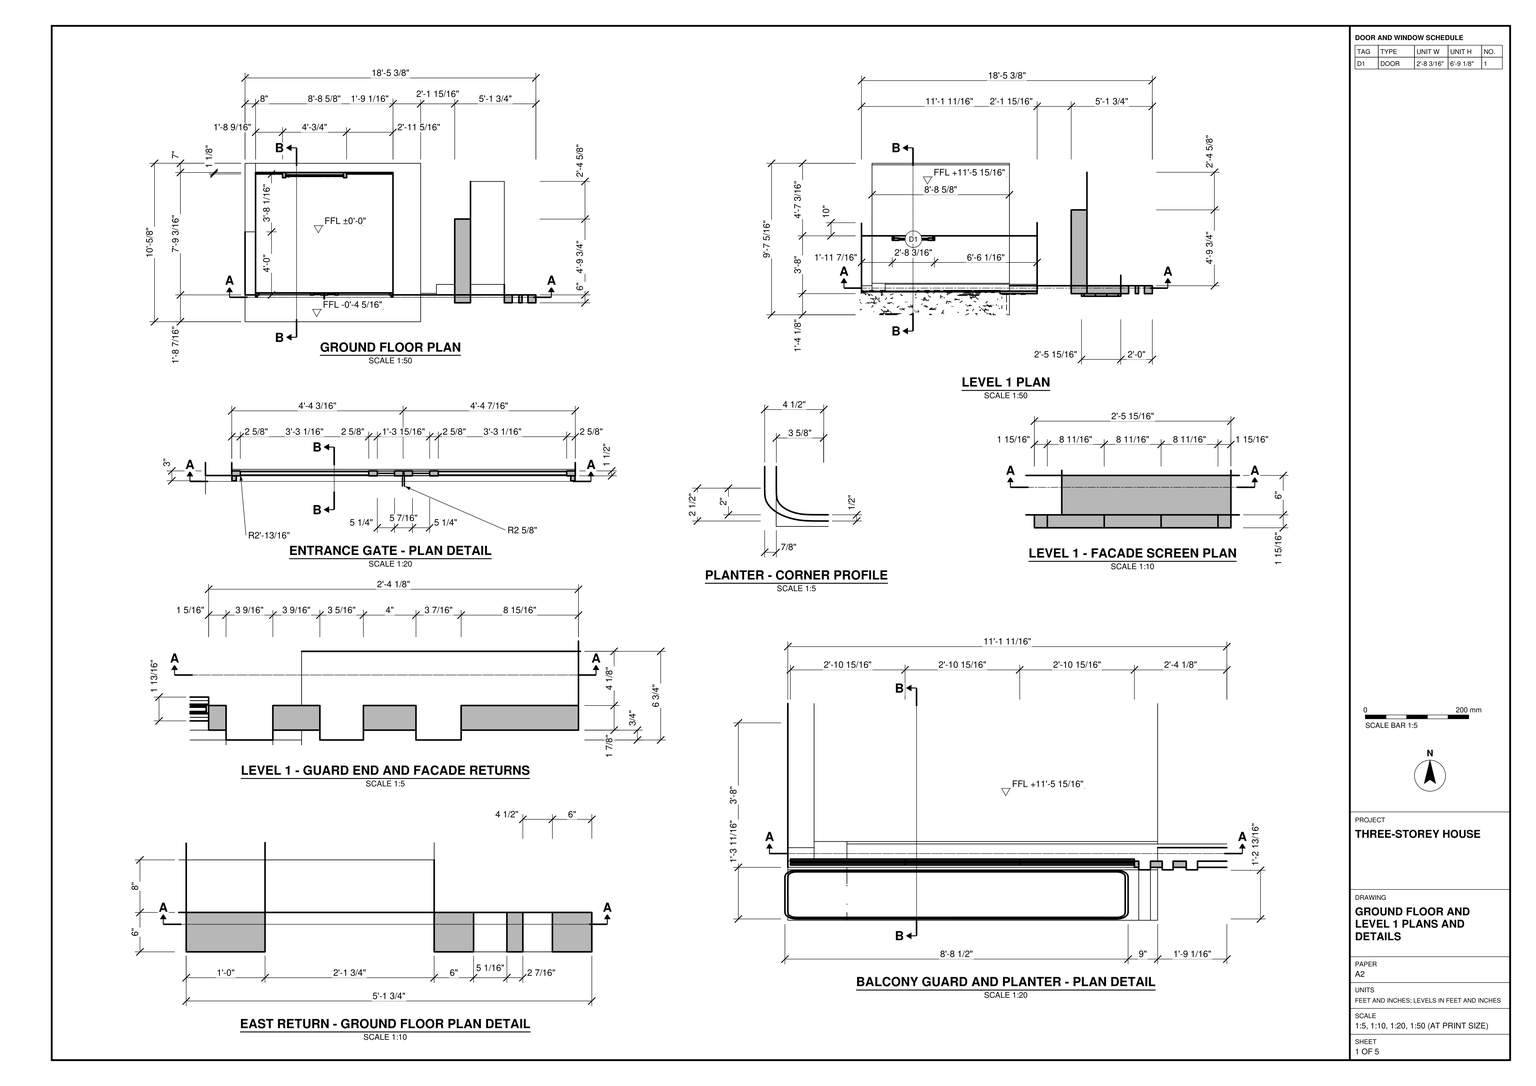
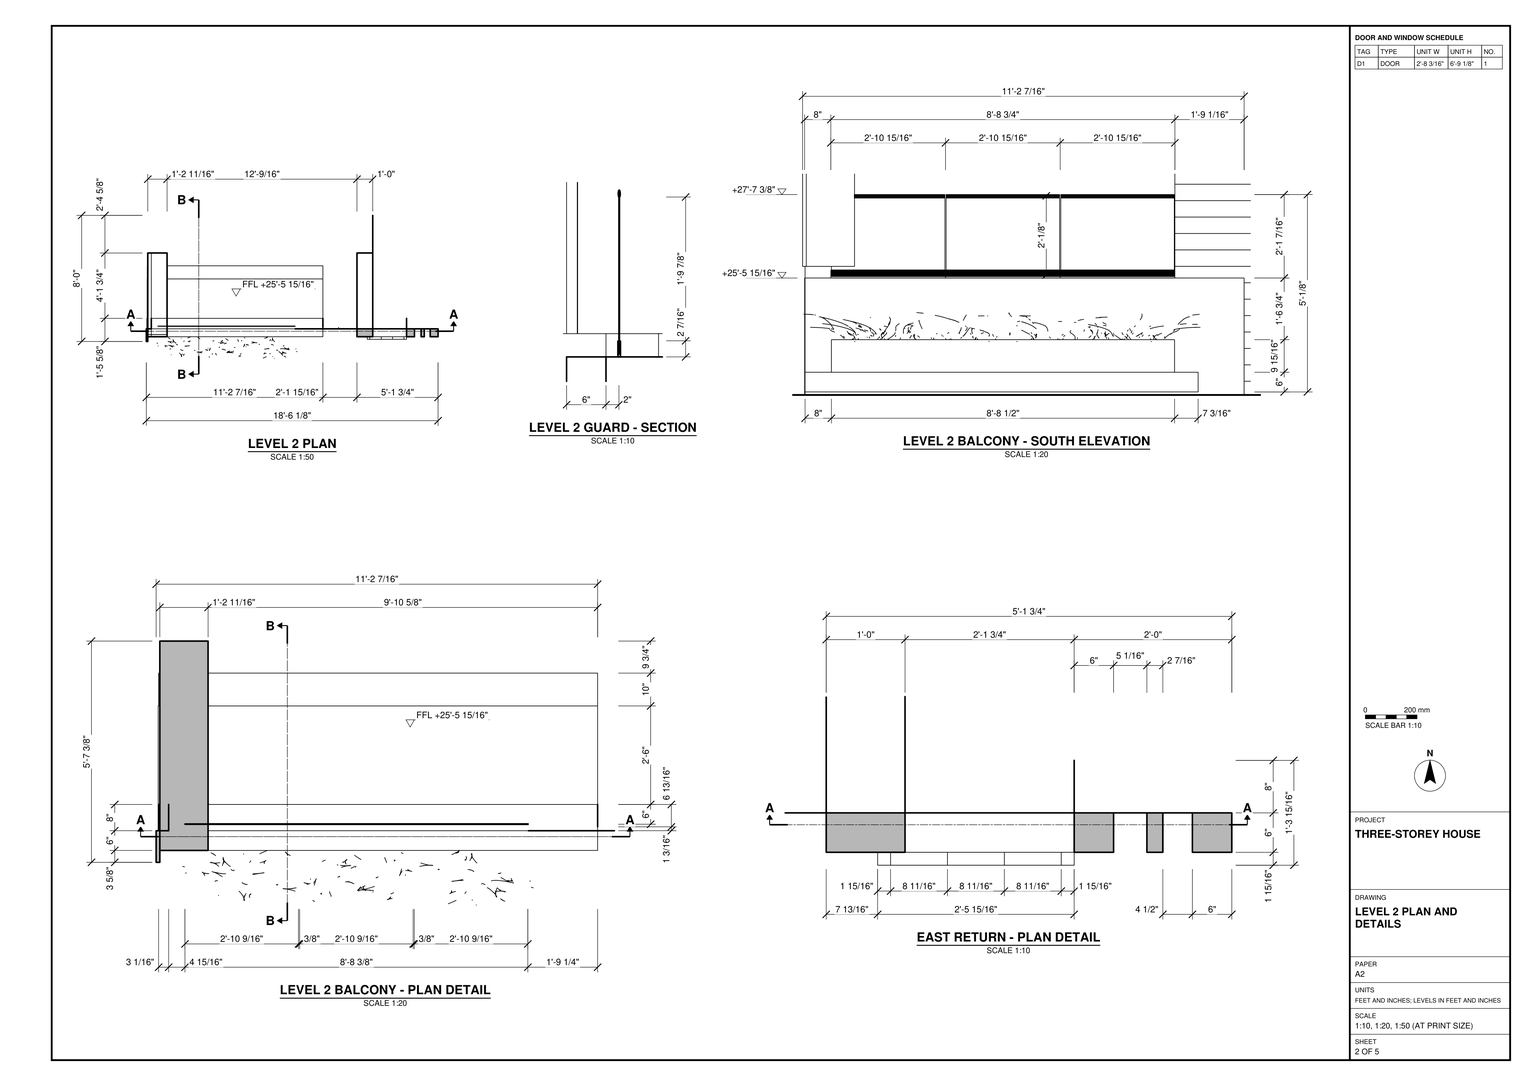
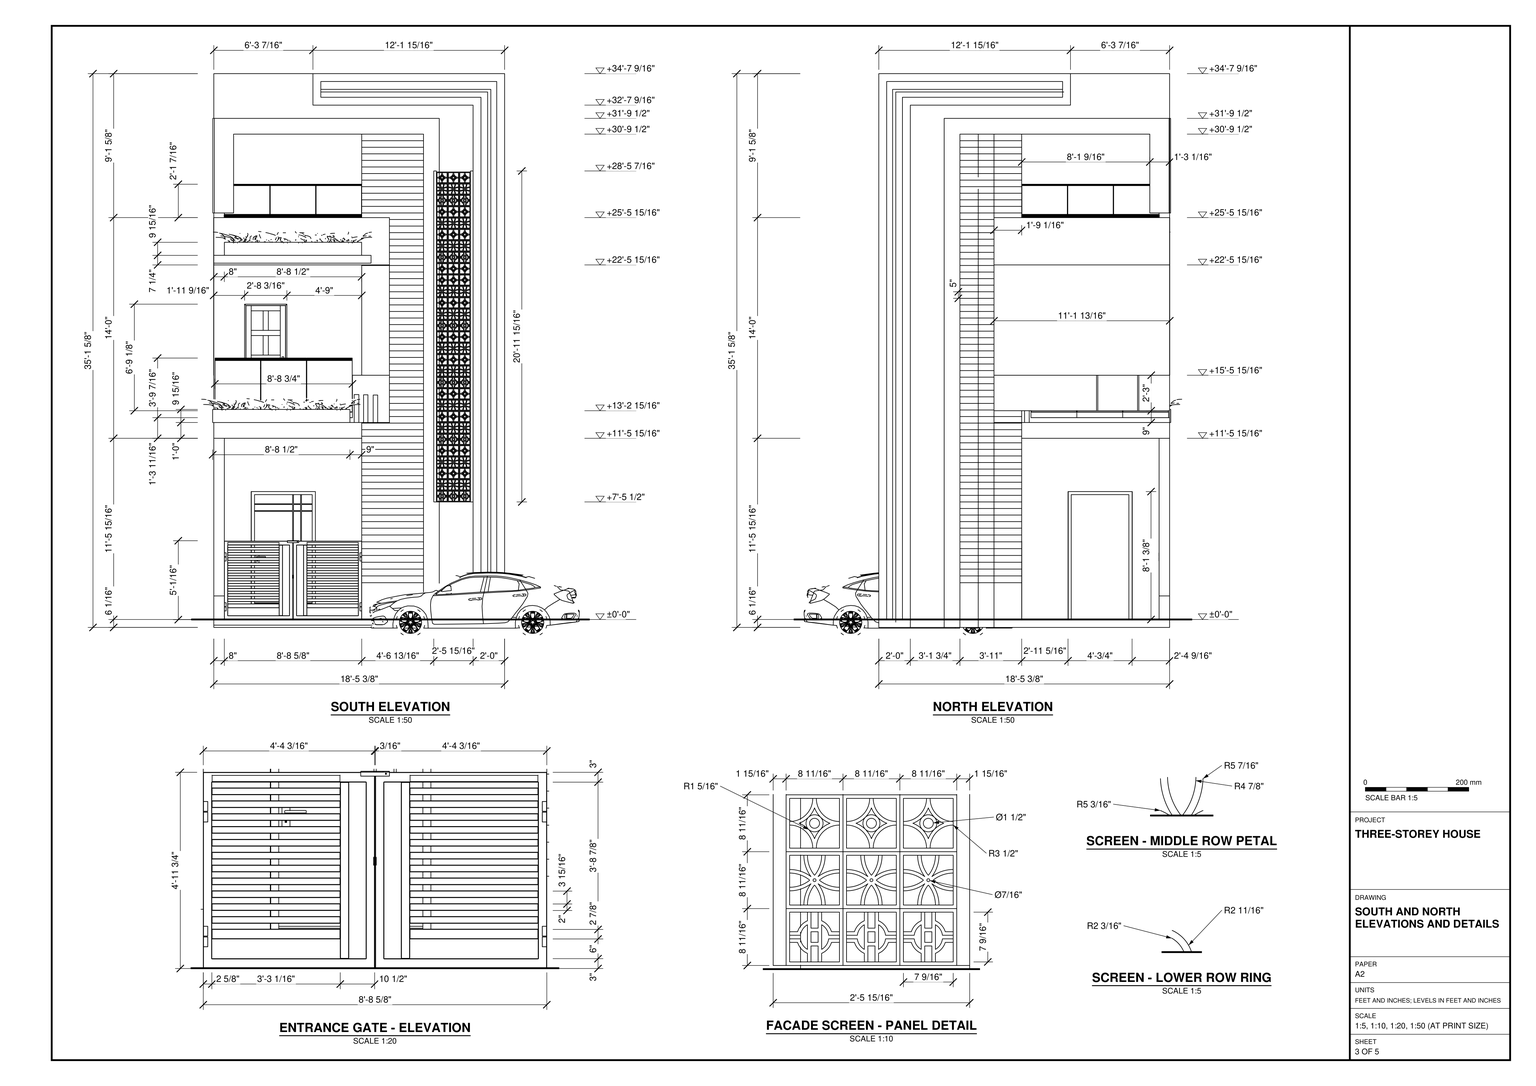
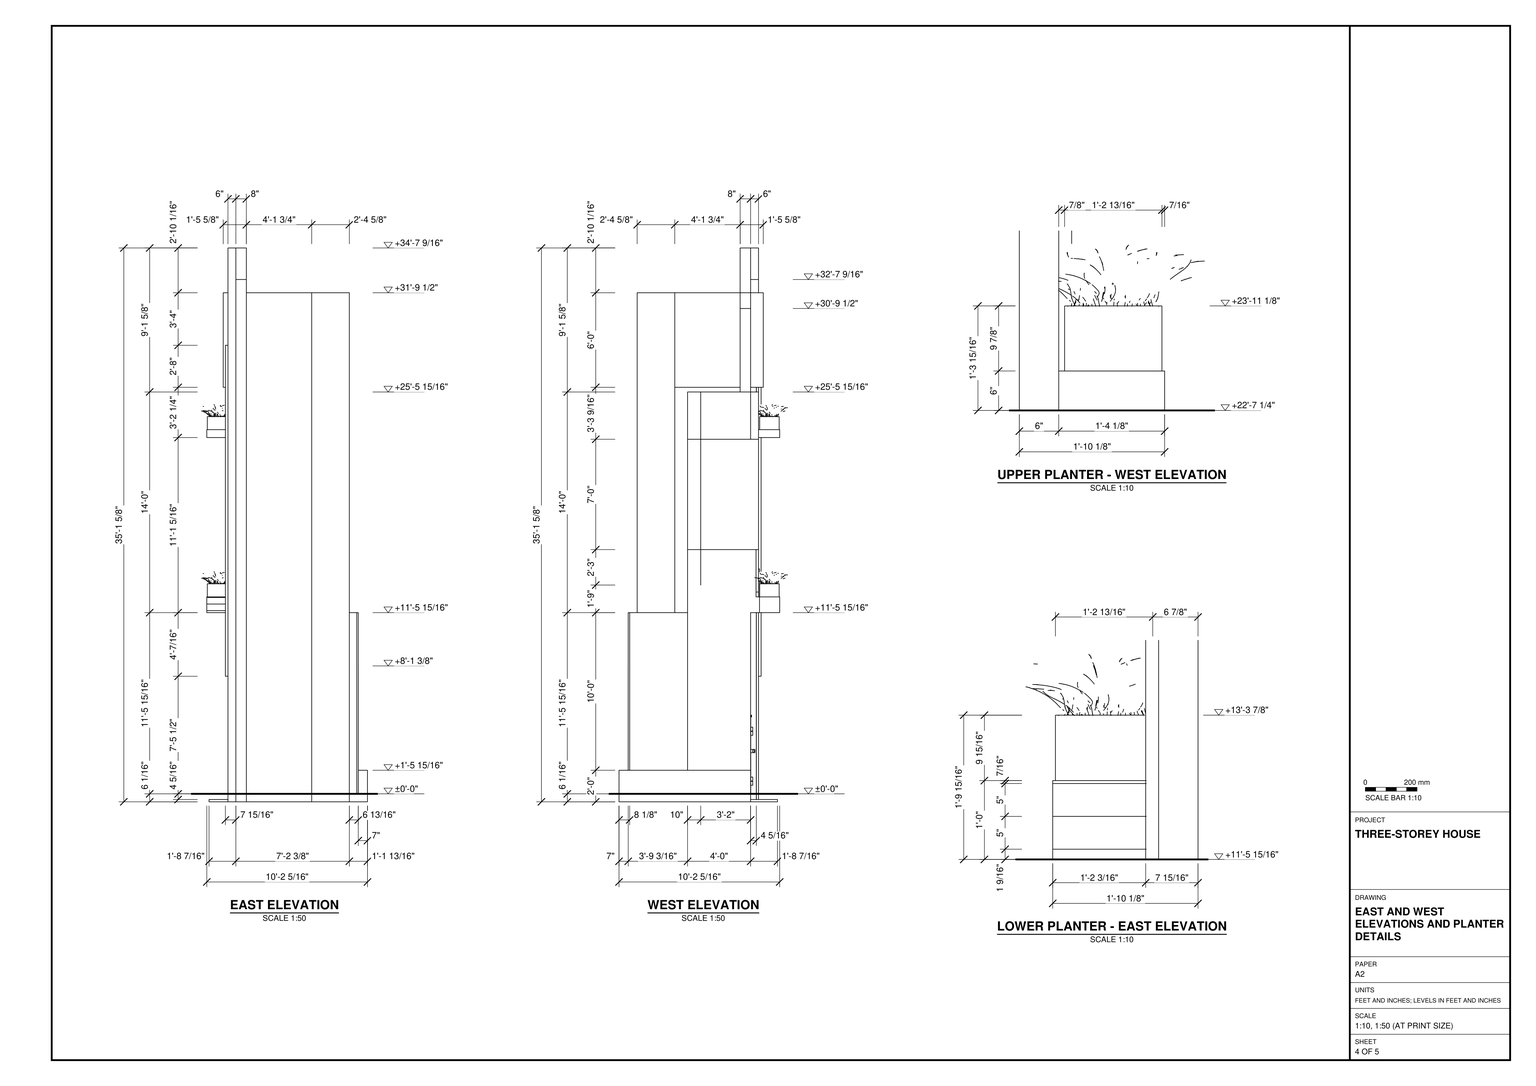
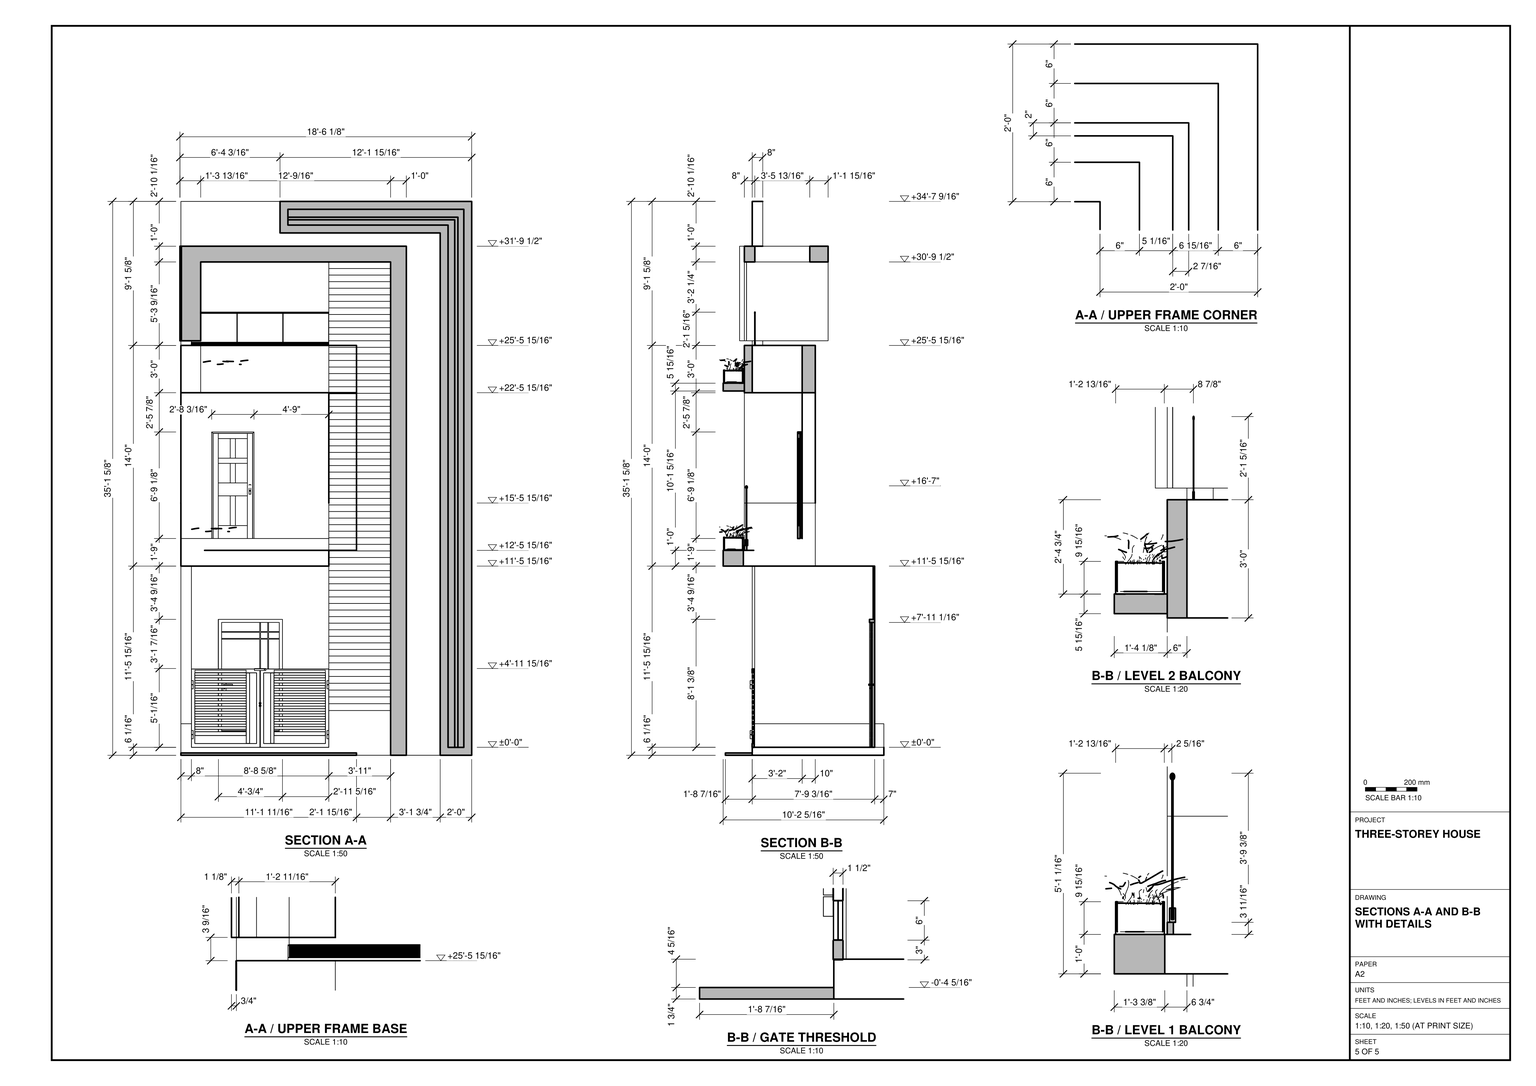
Build the three-storey house frontage in SketchUp from task_files/diagram_01.pdf. Work in feet and inches. The overall model extents, including the parked car, are 24'-11/16" along X, 17'-0" along Y and 35'-8 3/4" along Z. Set the finished floor levels to ±0'-0", +11'-5 15/16" and +25'-5 15/16".

Use the south elevation to lay out the entrance gate and stacked balconies on the left and the tall screened bay on the right. Use the plans and sections to give the walls their drawn thicknesses and to set the depths of the slabs, wall returns and roof-edge framing. Model the two framed, horizontally slatted gate leaves and the opening behind them. Place the scheduled door behind the lower balcony guard. Give both balconies panelled glass guards and projecting planter troughs, following the enlarged details for the guard ends, planter corners and supporting ledges.

Carry the horizontal wall courses alongside the balconies. Build the narrow patterned screen as openwork and continue the stepped outer frame across the top of the façade. Place the car beside the entrance as shown. Decor and loose items, including planting and the car, may be any suitable library components.

Keep walls, slabs, roof elements and individual furniture or joinery pieces in separate groups or components, and use components for repeated parts. Save one SketchUp model as output_files/three_storey_house_facade_with_balconies_and_gate.skp.

# SketchUp Ruby script. Lengths in inches.
U = 1.inch
M = Sketchup.active_model
def pt(a) = Geom::Point3d.new(a.map { |v| v * U })
def face(e, loops, mat)
  f = e.add_face(loops[0].map { |a| pt(a) })
  loops[1..].each { |l| e.add_face(l.map { |a| pt(a) }).erase! }
  f.material = f.back_material = mat if mat
  f
end
# faces: each face lists its corners as indices into pts; further lists are holes
def faces(e, pts, list, mat = nil) = list.each { |f| face(e, (f[0].is_a?(Array) ? f : [f]).map { |l| l.map { |i| pts[i] } }, mat) }
# xy, xz, yz: faces in a plane at the given z, y or x. An outline is a flat list of corners, or four numbers for a rectangle; further outlines are holes
def ring(l) = l.size == 4 ? [[l[0], l[1]], [l[2], l[1]], [l[2], l[3]], [l[0], l[3]]] : l.each_slice(2).to_a
def flat(e, list, mat, &to3) = list.each { |f| face(e, (f[0].is_a?(Array) ? f : [f]).map { |l| ring(l).map { |u, v| to3.(u, v) } }, mat) }
def xy(e, z, list, mat = nil) = flat(e, list, mat) { |x, y| [x, y, z] }
def xz(e, y, list, mat = nil) = flat(e, list, mat) { |x, z| [x, y, z] }
def yz(e, x, list, mat = nil) = flat(e, list, mat) { |y, z| [x, y, z] }
def lines(e, pts, list) = list.each { |a, b| e.add_line(pt(pts[a]), pt(pts[b])) }
# prism: a flat outline (further loops are holes) pulled along v
def prism(e, loops, v, mat = nil)
  f = face(e, loops, mat); d = Geom::Vector3d.new(v.map { |x| x * U })
  f.pushpull(f.normal.samedirection?(d) ? d.length : -d.length)
end
def box(e, o, s, mat = nil) = prism(e, [[o, [o[0] + s[0], o[1], o[2]], [o[0] + s[0], o[1] + s[1], o[2]], [o[0], o[1] + s[1], o[2]]]], [0, 0, s[2]], mat)
def at(x, y, z, deg = 0) = Geom::Transformation.translation(pt([x, y, z])) * Geom::Transformation.rotation(ORIGIN, Z_AXIS, deg.degrees)
def axes(o, x, y, z) = Geom::Transformation.new([*x, 0, *y, 0, *z, 0, *pt(o).to_a, 1])
def part(name) = M.definitions.add(name)
# library, detail: a bought-in or finely detailed component or shape, given as its bounding box
def library(name, o, s) = part(name).tap { |d| box(d.entities, o, s) }
def detail(e, o, s) = box(e.add_group.entities, o, s)
def put(e, d, t, mat = nil) = e.add_instance(d, t).tap { |i| i.material = mat if mat }
def group(e, t, mat = nil) = e.add_group.tap { |g| g.transformation = t; g.material = mat if mat }.entities
root = M.entities
M.materials.add("[0092_Azure]").color = [240, 255, 255]
M.materials.add("[0110_LightSlateGray]").color = [119, 136, 153]
M.materials.add("[0134_DimGray]").color = [105, 105, 105]
M.materials.add("[0135_DarkGray]").color = [81, 81, 81]
M.materials.add("[Cladding Siding Tan]").color = [162, 126, 95]
M.materials.add("[Color D06]").color = [204, 80, 30]
M.materials.add("[Field Square Tile]").color = [217, 201, 169]
M.materials.add("[Tile Limestone Multi]").color = [199, 173, 118]
c1 = library("Residential Interior Door",[0,-1.69,0],[32.2,5.15,81.1])
c2 = library("Untitled",[0,0,0],[36,4.39,84])
c3 = library("T1",[0,0,0],[8.66,8.66,1.97])
c4 = library("T2",[0,0,0],[8.66,8.66,1.97])
c5 = library("T3",[0,0,0],[8.66,8.66,1.97])
c6 = part("1")
box(c6.entities,[-1.97,0,0],[1.97,251.97,1.97],"[0134_DimGray]")
box(c6.entities,[25.98,0,0],[1.97,251.97,1.97],"[0134_DimGray]")
put(c6.entities,c3,at(0,43.31,0),"[Color D06]")
put(c6.entities,c4,at(17.32,25.98,0),"[Color D06]")
put(c6.entities,c5,at(0,34.65,0),"[Color D06]")
put(c6.entities,c4,at(0,8.66,0),"[Color D06]")
put(c6.entities,c5,at(8.66,34.65,0),"[Color D06]")
put(c6.entities,c3,at(8.66,43.31,0),"[Color D06]")
put(c6.entities,c4,at(0,25.98,0),"[Color D06]")
put(c6.entities,c5,at(17.32,34.65,0),"[Color D06]")
put(c6.entities,c4,at(8.66,25.98,0),"[Color D06]")
put(c6.entities,c5,at(17.32,147.24,0),"[Color D06]")
put(c6.entities,c4,at(0,51.97,0),"[Color D06]")
put(c6.entities,c3,at(0,0,0),"[Color D06]")
put(c6.entities,c5,at(8.66,147.24,0),"[Color D06]")
put(c6.entities,c3,at(8.66,0,0),"[Color D06]")
put(c6.entities,c5,at(17.32,17.32,0),"[Color D06]")
put(c6.entities,c4,at(17.32,8.66,0),"[Color D06]")
put(c6.entities,c5,at(8.66,17.32,0),"[Color D06]")
put(c6.entities,c5,at(0,17.32,0),"[Color D06]")
put(c6.entities,c3,at(17.32,0,0),"[Color D06]")
put(c6.entities,c4,at(8.66,8.66,0),"[Color D06]")
put(c6.entities,c3,at(17.32,43.31,0),"[Color D06]")
put(c6.entities,c4,at(8.66,51.97,0),"[Color D06]")
put(c6.entities,c5,at(0,121.26,0),"[Color D06]")
put(c6.entities,c3,at(0,129.92,0),"[Color D06]")
put(c6.entities,c3,at(8.66,129.92,0),"[Color D06]")
put(c6.entities,c4,at(17.32,138.58,0),"[Color D06]")
put(c6.entities,c5,at(0,60.63,0),"[Color D06]")
put(c6.entities,c5,at(8.66,121.26,0),"[Color D06]")
put(c6.entities,c5,at(17.32,121.26,0),"[Color D06]")
put(c6.entities,c4,at(0,112.6,0),"[Color D06]")
put(c6.entities,c4,at(8.66,112.6,0),"[Color D06]")
put(c6.entities,c5,at(8.66,60.63,0),"[Color D06]")
put(c6.entities,c5,at(17.32,60.63,0),"[Color D06]")
put(c6.entities,c4,at(17.32,51.97,0),"[Color D06]")
put(c6.entities,c4,at(17.32,112.6,0),"[Color D06]")
put(c6.entities,c5,at(0,147.24,0),"[Color D06]")
put(c6.entities,c4,at(17.32,69.29,0),"[Color D06]")
put(c6.entities,c5,at(8.66,77.95,0),"[Color D06]")
put(c6.entities,c5,at(0,77.95,0),"[Color D06]")
put(c6.entities,c3,at(8.66,86.61,0),"[Color D06]")
put(c6.entities,c5,at(17.32,77.95,0),"[Color D06]")
put(c6.entities,c4,at(8.66,95.28,0),"[Color D06]")
put(c6.entities,c4,at(8.66,69.29,0),"[Color D06]")
put(c6.entities,c3,at(0,86.61,0),"[Color D06]")
put(c6.entities,c3,at(17.32,86.61,0),"[Color D06]")
put(c6.entities,c5,at(0,103.9375,0),"[Color D06]")
put(c6.entities,c5,at(8.66,103.9375,0),"[Color D06]")
put(c6.entities,c5,at(17.32,103.9375,0),"[Color D06]")
put(c6.entities,c4,at(0,95.28,0),"[Color D06]")
put(c6.entities,c4,at(0,69.29,0),"[Color D06]")
put(c6.entities,c4,at(17.32,95.28,0),"[Color D06]")
put(c6.entities,c5,at(8.66,164.57,0),"[Color D06]")
put(c6.entities,c5,at(0,164.57,0),"[Color D06]")
put(c6.entities,c5,at(17.32,199.21,0),"[Color D06]")
put(c6.entities,c3,at(0,181.89,0),"[Color D06]")
put(c6.entities,c4,at(17.32,190.55,0),"[Color D06]")
put(c6.entities,c3,at(8.66,181.89,0),"[Color D06]")
put(c6.entities,c3,at(17.32,181.89,0),"[Color D06]")
put(c6.entities,c5,at(17.32,164.57,0),"[Color D06]")
put(c6.entities,c5,at(0,199.21,0),"[Color D06]")
put(c6.entities,c5,at(8.66,173.23,0),"[Color D06]")
put(c6.entities,c5,at(8.66,199.21,0),"[Color D06]")
put(c6.entities,c5,at(17.32,173.23,0),"[Color D06]")
put(c6.entities,c4,at(8.66,155.91,0),"[Color D06]")
put(c6.entities,c4,at(0,190.55,0),"[Color D06]")
put(c6.entities,c4,at(8.66,190.55,0),"[Color D06]")
put(c6.entities,c4,at(0,155.91,0),"[Color D06]")
put(c6.entities,c4,at(17.32,155.91,0),"[Color D06]")
put(c6.entities,c5,at(0,173.23,0),"[Color D06]")
put(c6.entities,c4,at(8.66,207.875,0),"[Color D06]")
put(c6.entities,c4,at(0,233.86,0),"[Color D06]")
put(c6.entities,c4,at(8.66,233.86,0),"[Color D06]")
put(c6.entities,c4,at(0,138.58,0),"[Color D06]")
put(c6.entities,c3,at(17.32,129.92,0),"[Color D06]")
put(c6.entities,c5,at(0,216.53,0),"[Color D06]")
put(c6.entities,c3,at(8.66,225.2,0),"[Color D06]")
put(c6.entities,c4,at(17.32,207.875,0),"[Color D06]")
put(c6.entities,c4,at(17.32,233.86,0),"[Color D06]")
put(c6.entities,c5,at(8.66,242.52,0),"[Color D06]")
put(c6.entities,c4,at(0,207.875,0),"[Color D06]")
put(c6.entities,c4,at(8.66,138.58,0),"[Color D06]")
put(c6.entities,c5,at(17.32,216.53,0),"[Color D06]")
put(c6.entities,c5,at(8.66,216.53,0),"[Color D06]")
put(c6.entities,c5,at(17.32,242.52,0),"[Color D06]")
put(c6.entities,c3,at(17.32,225.2,0),"[Color D06]")
put(c6.entities,c5,at(0,242.52,0),"[Color D06]")
put(c6.entities,c3,at(0,225.2,0),"[Color D06]")
c7 = library("2016+Honda+Civic+LX+Sedan",[0.01,0.03,0.02],[16.17,34.46,10.62])
c8 = library("Wagner Glass Railing",[9.08,102.375,1.53],[2.51,145.5,42.05])
c9 = library("Group13",[-203.48,36.63,0],[29.68,67.31,50.64])
c10 = library("Group\#1076",[0,-1.74,0],[119.75,5.32,60.06])
xy(root,16.53,[[0.75,1.6875,134.4375,22.125],[160.375,16.125,172.375,17.75],[198.125,16.125,222.125,22.125],[160.375,17.75,172.375,17.8125],[160.375,17.8125,172.375,22.125],
  [0.75,22.125,134.4375,122.3125],[134.4375,22.125,146.4375,23.3125],[146.4375,22.125,160.375,30.125],[160.375,22.125,172.375,30.125],[172.375,22.125,198.125,30.125],
  [160.375,30.125,172.375,79.875],[172.375,30.125,198.125,108.5]])
xy(root,18.28,[[0.75,1.6875,134.4375,22.125]])
xy(root,22.53,[[204.125,16.125,209.2,22.125],[209.2,16.125,211.625,22.125],[211.625,16.125,216.125,22.125]])
xy(root,22.59,[[8.75,22.125,113.36,24],[8.75,24,113.36,24,113.36,114.1875,77.9,114.1875,77.9,115.3125,29.15,115.3125,29.15,114.1875,8.75,114.1875],[8.75,114.1875,29.15,115.3125],[77.9,114.1875,113.36,115.3125]])
xy(root,40.53,[[0.75,22.125,8.75,70.125],[0.75,70.125,8.75,122.3125]])
xy(root,119.97,[[29.15,114.1875,77.9,115.3125]])
xy(root,160.53,[[0.75,0,8.75,15.375],[8.75,0,18.75,15.375],[18.75,0,113.36,15.375],[0.75,15.375,8.75,22.125],[8.75,15.375,18.75,24],
  [18.75,15.375,113.36,24],[8.75,24,113.36,114.1875],[8.75,114.1875,113.36,115.3125]])
xy(root,172.53,[[0.75,0,18.75,15.375],[18.75,0,107.61,15.375],[107.61,0,111.17,15.375],[111.17,0,113.36,15.375],[0.75,15.375,18.75,16.125],
  [107.61,15.375,111.17,15.375,111.17,18,113.36,18,113.36,22.125,134.4375,22.125,134.4375,23.25,18.75,23.25,18.75,18,107.61,18],[18.75,15.375,107.61,16.125],[111.17,15.375,113.36,16.125],[114.75,15.375,114.75,18,113.36,18,113.36,22.125,134.4375,22.125,134.4375,18,125.5,18,125.5,15.375,122.07,15.375,122.07,18,118.06,18,118.06,15.375],[111.17,16.125,113.36,18],
  [113.36,16.125,114.75,18],[118.06,16.125,122.07,18]])
xy(root,172.53,[[0.75,16.125,18.75,18],[18.75,16.125,107.61,18],[125.5,16.125,134.4375,18]],"[0135_DarkGray]")
xy(root,176.22,[[0.75,16.125,106.28,18]],"[0135_DarkGray]")
xy(root,193.47,[[122.07,15.375,125.5,16.125]],"[0092_Azure]")
xy(root,193.47,[[122.07,16.125,125.5,18]],"[0135_DarkGray]")
xy(root,193.65,[[114.75,15.375,118.06,16.125]],"[0092_Azure]")
xy(root,193.65,[[114.75,16.125,118.06,18]],"[0135_DarkGray]")
xy(root,193.84,[[107.61,15.375,111.17,16.125]],"[0092_Azure]")
xy(root,193.84,[[107.61,16.125,111.17,18]],"[0135_DarkGray]")
xy(root,208.53,[[0.625,16.125,0.625,60.125,0.75,16.125],[0.75,16.125,0.625,60.125,0.75,60.125]])
xy(root,208.53,[[106.28,16.125,113.36,18],[113.36,16.125,134.4375,18]],"[0135_DarkGray]")
xy(root,292.08,[[113.36,16.125,134.4375,22.125]])
xy(root,292.53,[[0.75,16.125,0.73,22.125,0.75,22.125],[0.75,16.125,134.4375,22.125],[0.625,22.125,0.625,60.125,0.73,22.125],[0.75,60.125,134.4375,70.125]])
xy(root,292.53,[[0.73,22.125,0.625,60.125,134.4375,60.125,134.4375,22.125]],"[Field Square Tile]")
xy(root,293.83,[[0.75,0,120.4375,16.125]],"[0092_Azure]")
xy(root,299.83,[[0.75,0,120.4375,16.125]],"[0092_Azure]")
xy(root,328.53,[[0.75,16.125,134.4375,22.125],[0.625,22.125,0.75,22.125,0.75,30.125,15.8125,30.125,15.8125,60.125,0.625,60.125],[0.75,22.125,15.8125,30.125],[15.8125,22.125,134.4375,30.125],[15.8125,30.125,134.4375,60.125],
  [0.75,60.125,134.4375,70.125]])
xy(root,332.07,[[0,12.5,1.125,22.125],[1.125,16.125,3.8125,17.75],[3.8125,16.125,15.8125,17.75],[1.125,17.75,3.8125,17.8125],[3.8125,17.75,15.8125,17.8125],
  [1.125,17.8125,3.8125,22.125],[3.8125,17.8125,15.8125,22.125],[1.125,22.125,3.8125,79.875],[3.8125,22.125,15.8125,30.125],[3.8125,30.125,15.8125,79.875]])
xy(root,392.08,[[15.8125,16.125,18.75,17.75],[[18.75,16.125,18.75,79.875,160.375,79.875,160.375,22.125,146.4375,22.125,146.4375,23.3125,134.4375,23.3125,134.4375,22.125,160.375,22.125,160.375,16.125],[29.05,24.12,43.55,65.93],[50.19,23.69,63.07,65.69]],[15.8125,17.75,18.75,17.8125],[15.8125,17.8125,18.75,22.125],[15.8125,22.125,18.75,30.125],
  [134.4375,22.125,146.4375,23.3125],[134.4375,22.125,146.4375,23.3125],[15.8125,30.125,18.75,79.875]])
xy(root,404.07,[[0,12.5,1.125,22.125],[1.125,16.125,146.4375,17.75],[146.4375,16.125,172.375,17.75],[1.125,17.75,146.4375,17.8125],[146.4375,17.75,172.375,17.8125],
  [1.125,17.8125,146.4375,22.125],[146.4375,17.8125,172.375,22.125],[1.125,22.125,3.8125,79.875],[3.8125,22.125,18.75,30.125],[3.8125,22.125,18.75,79.875],
  [18.75,22.125,146.4375,22.125,146.4375,30.125,63.07,30.125,63.07,23.69,50.19,23.69,50.19,30.125,43.55,30.125,43.55,24.12,29.05,24.12,29.05,30.125,18.75,30.125],[146.4375,22.125,172.375,79.875],[50.19,23.69,63.07,30.125],[29.05,24.12,43.55,30.125],[3.8125,30.125,18.75,79.875],
  [18.75,30.125,29.05,30.125,29.05,65.93,43.55,65.93,43.55,30.125,50.19,30.125,50.19,65.69,63.07,65.69,63.07,30.125,146.4375,30.125,146.4375,79.875,18.75,79.875],[146.4375,79.875,172.375,108.5]])
xy(root,414.15,[[76.22,16.125,198.125,22.125],[76.22,22.125,198.125,30.125]])
xy(root,420.15,[[82.22,16.125,204.125,22.125]],"[0110_LightSlateGray]")
xy(root,424.17,[[82.22,16.125,209.2,22.125]],"[0110_LightSlateGray]")
xy(root,426.15,[[82.22,16.125,211.625,22.125]],"[0110_LightSlateGray]")
xy(root,432.15,[[82.22,16.125,216.125,22.125]])
xy(root,438.15,[[76.22,16.125,222.125,22.125],[0.75,22.125,76.22,30.125]])
xz(root,0,[[0.75,160.53,113.36,172.53]])
xz(root,0,[[0.75,293.83,120.4375,299.83]],"[0092_Azure]")
xz(root,1.6875,[[0.75,16.53,134.4375,18.28]])
xz(root,12.5,[[0,332.07,1.125,404.07]])
xz(root,15.375,[[0.75,160.53,113.36,172.53]])
xz(root,15.375,[[107.61,172.53,111.17,193.84],[114.75,172.53,118.06,193.65],[122.07,172.53,125.5,193.47]],"[0092_Azure]")
xz(root,16.125,[[160.375,16.53,172.375,16.53,172.375,404.07,1.125,404.07,1.125,332.07,15.8125,332.07,15.8125,392.08,160.375,392.08],[209.2,22.53,211.625,22.53,211.625,426.15,82.22,426.15,82.22,424.17,209.2,424.17]])
xz(root,16.125,[[0.75,293.83,120.4375,299.83]],"[0092_Azure]")
xz(root,16.125,[[[198.125,16.53,222.125,16.53,222.125,438.15,76.22,438.15,76.22,414.15,198.125,414.15],[204.125,22.53,204.125,420.15,82.22,420.15,82.22,432.15,216.125,432.15,216.125,22.53]]],"[0110_LightSlateGray]")
xz(root,16.125,[[0.75,172.53,107.61,172.53,107.61,193.84,111.17,193.84,111.17,172.53,114.75,172.53,114.75,193.65,118.06,193.65,118.06,172.53,122.07,172.53,122.07,193.47,125.5,193.47,125.5,172.53,134.4375,172.53,134.4375,208.53,106.28,208.53,106.28,176.22,0.75,176.22],[113.36,208.53,134.4375,292.08],[0.75,292.53,134.4375,292.53,134.4375,328.53,0.75,328.53,0.75,299.83,120.4375,299.83,120.4375,293.83,0.75,293.83]],"[0135_DarkGray]")
xz(root,18,[[0.75,172.53,0.75,176.22,106.28,176.22,106.28,208.53,134.4375,208.53,134.4375,172.53,125.5,172.53,125.5,193.47,122.07,193.47,122.07,172.53,118.06,172.53,118.06,193.65,114.75,193.65,114.75,172.53,111.17,172.53,111.17,193.84,107.61,193.84,107.61,172.53]],"[0135_DarkGray]")
xz(root,22.125,[[0.75,16.53,134.4375,18.28],[134.4375,16.53,160.375,16.53,160.375,50.58,113.36,50.58,113.36,22.59,8.75,22.59,8.75,40.53,0.75,40.53,0.75,18.28,134.4375,18.28],[[198.125,16.53,198.125,414.15,76.22,414.15,76.22,438.15,222.125,438.15,222.125,16.53],[204.125,22.53,216.125,22.53,216.125,432.15,82.22,432.15,82.22,420.15,204.125,420.15]],[160.375,16.53,172.375,16.53,172.375,404.07,146.4375,404.07,146.4375,392.08,160.375,392.08],[209.2,22.53,209.2,424.17,82.22,424.17,82.22,426.15,211.625,426.15,211.625,22.53],
  [0.75,40.53,8.75,160.53],[113.36,50.58,160.375,55.77],[113.36,172.08,134.4375,172.53],[113.36,172.53,134.4375,177.08],[113.36,177.08,134.4375,182.08],
  [113.36,182.08,134.4375,187.08],[113.36,187.08,134.4375,192.08],[113.36,192.08,134.4375,197.08],[113.36,197.08,134.4375,202.08],[113.36,202.08,134.4375,207.08],
  [113.36,207.08,134.4375,212.08],[113.36,212.08,134.4375,217.08],[113.36,217.08,134.4375,222.08],[113.36,222.08,134.4375,227.08],[113.36,227.08,134.4375,232.08],
  [113.36,232.08,134.4375,237.08],[113.36,237.08,134.4375,242.08],[113.36,242.08,134.4375,247.08],[113.36,247.08,134.4375,252.08],[113.36,252.08,134.4375,257.08],
  [113.36,257.08,134.4375,262.08],[113.36,262.08,134.4375,267.08],[113.36,267.08,134.4375,272.08],[113.36,272.08,134.4375,277.08],[113.36,277.08,134.4375,282.08],
  [113.36,282.08,134.4375,287.08],[113.36,287.08,134.4375,292.08],[113.36,292.08,134.4375,292.53],[0.625,292.53,0.75,328.53],[0.75,292.53,15.8125,328.53],
  [15.8125,292.53,113.36,328.53],[113.36,292.53,134.4375,297.08],[113.36,297.08,134.4375,302.08],[113.36,302.08,134.4375,307.08],[113.36,307.08,134.4375,312.08],
  [113.36,312.08,134.4375,317.08],[113.36,317.08,134.4375,322.08],[113.36,322.08,134.4375,327.08],[113.36,327.08,134.4375,328.53],[0,332.07,0.75,404.07],
  [0.75,332.07,1.125,404.07],[1.125,332.07,3.8125,404.07]])
xz(root,22.125,[[204.125,22.53,209.2,22.53,209.2,424.17,82.22,424.17,82.22,420.15,204.125,420.15],[211.625,22.53,216.125,22.53,216.125,432.15,82.22,432.15,82.22,426.15,211.625,426.15]],"[0110_LightSlateGray]")
xz(root,22.125,[[113.36,55.77,160.375,60.96],[113.36,60.96,160.375,66.15],[113.36,66.15,160.375,71.33],[113.36,71.33,160.375,76.52],[113.36,76.52,160.375,81.71],
  [113.36,81.71,160.375,86.9],[113.36,86.9,160.375,92.08],[113.36,92.08,160.375,97.08],[113.36,97.08,160.375,102.08],[113.36,102.08,160.375,107.08],
  [113.36,107.08,160.375,112.08],[113.36,112.08,160.375,117.08],[113.36,117.08,160.375,122.08],[113.36,122.08,160.375,127.08],[113.36,127.08,160.375,132.08],
  [113.36,132.08,160.375,137.08],[113.36,137.08,160.375,142.08],[113.36,142.08,160.375,147.08],[113.36,147.08,160.375,152.08],[113.36,152.08,160.375,157.08],
  [113.36,157.08,160.375,162.08],[113.36,162.08,160.375,167.08],[113.36,167.08,160.375,172.08],[134.4375,172.08,160.375,177.08],[134.4375,177.08,160.375,182.08],
  [134.4375,182.08,160.375,187.08],[134.4375,187.08,160.375,192.08],[134.4375,192.08,160.375,197.08],[134.4375,197.08,160.375,202.08],[134.4375,202.08,160.375,207.08],
  [134.4375,207.08,160.375,212.08],[134.4375,212.08,160.375,217.08],[134.4375,217.08,160.375,222.08],[134.4375,222.08,160.375,227.08],[134.4375,227.08,160.375,232.08],
  [134.4375,232.08,160.375,237.08],[134.4375,237.08,160.375,242.08],[134.4375,242.08,160.375,247.08],[134.4375,247.08,160.375,252.08],[134.4375,252.08,160.375,257.08],
  [134.4375,257.08,160.375,262.08],[134.4375,262.08,160.375,267.08],[134.4375,267.08,160.375,272.08],[134.4375,272.08,160.375,277.08],[134.4375,277.08,160.375,282.08],
  [134.4375,282.08,160.375,287.08],[134.4375,287.08,160.375,292.08],[134.4375,292.08,160.375,297.08],[134.4375,297.08,160.375,302.08],[134.4375,302.08,160.375,307.08],
  [134.4375,307.08,160.375,312.08],[134.4375,312.08,160.375,317.08],[134.4375,317.08,160.375,322.08],[134.4375,322.08,160.375,327.08],[134.4375,327.08,160.375,327.08,160.375,332.08,113.36,332.08,113.36,328.53,134.4375,328.53],
  [113.36,332.08,160.375,337.08],[113.36,337.08,160.375,342.08],[113.36,342.08,160.375,347.08],[113.36,347.08,160.375,352.08],[113.36,352.08,160.375,357.08],
  [113.36,357.08,160.375,362.08],[113.36,362.08,160.375,367.08],[113.36,367.08,160.375,372.08],[113.36,372.08,160.375,377.08],[113.36,377.08,160.375,382.08],
  [113.36,382.08,160.375,387.08],[113.36,387.08,160.375,392.08]],"[Cladding Siding Tan]")
xz(root,22.125,[[172.375,16.53,198.125,16.53,198.125,414.15,76.22,414.15,76.22,438.15,0.75,438.15,0.75,404.07,172.375,404.07]],"[Tile Limestone Multi]")
xz(root,23.69,[[50.19,392.08,63.07,404.07]])
xz(root,24.12,[[29.05,392.08,43.55,404.07]])
xz(root,60.125,[[0.625,208.53,0.75,280.15],[0.625,280.15,0.75,291.09],[0.625,291.09,0.75,292.53],[0.625,292.53,0.75,328.53],[0.75,292.53,15.8125,328.53],
  [15.8125,292.53,134.4375,328.53]])
xz(root,60.125,[[0.75,181.53,134.4375,292.53]],"[Field Square Tile]")
xz(root,65.69,[[50.19,392.08,63.07,404.07]])
xz(root,65.93,[[29.05,392.08,43.55,404.07]])
xz(root,70.125,[[0.75,208.53,134.4375,292.53],[0.75,292.53,134.4375,328.53]])
xz(root,79.875,[[160.375,16.53,160.375,392.08,15.8125,392.08,15.8125,332.07,1.125,332.07,1.125,404.07,172.375,404.07,172.375,16.53]])
xz(root,114.1875,[[8.75,22.59,29.15,22.59,29.15,119.97,77.9,119.97,77.9,22.59,113.36,22.59,113.36,160.53,8.75,160.53]],"[Field Square Tile]")
xz(root,115.3125,[[8.75,22.59,8.75,160.53,113.36,160.53,113.36,22.59,77.9,22.59,77.9,119.97,29.15,119.97,29.15,22.59],[29.15,22.59,77.9,119.97]])
xz(root,122.3125,[[0.75,16.53,0.75,40.53,8.75,40.53,8.75,22.59,134.4375,22.59,134.4375,16.53]])
yz(root,0,[[12.5,332.07,22.125,404.07]])
yz(root,0.625,[[22.125,292.53,60.125,328.53]])
yz(root,0.75,[[1.6875,16.53,22.125,18.28],[22.125,16.53,122.3125,40.53],[22.125,40.53,22.125,160.53,15.375,160.53,15.375,172.53,18,172.53,18,208.53,70.125,208.53,70.125,40.53],[0,160.53,15.375,172.53],[60.125,208.53,70.125,292.53],
  [16.125,292.53,22.125,328.53],[60.125,292.53,70.125,328.53],[22.125,328.53,30.125,392.08],[22.125,392.08,30.125,404.07],[22.125,404.07,30.125,438.15]])
yz(root,0.75,[[0,293.83,16.125,299.83]],"[0092_Azure]")
yz(root,0.75,[[16.125,172.53,18,176.22],[16.125,176.22,18,208.53]],"[0135_DarkGray]")
yz(root,1.125,[[12.5,332.07,16.125,404.07],[16.125,332.07,17.75,404.07],[17.75,332.07,17.8125,404.07],[17.8125,332.07,22.125,404.07],[22.125,332.07,79.875,404.07]])
yz(root,3.8125,[[22.125,332.07,30.125,404.07]])
yz(root,8.75,[[22.125,22.59,24,40.53],[24,22.59,114.1875,40.53],[114.1875,22.59,115.3125,40.53],[115.3125,22.59,122.3125,40.53],[22.125,40.53,24,160.53],
  [114.1875,40.53,115.3125,160.53]])
yz(root,8.75,[[24,40.53,114.1875,160.53]],"[Field Square Tile]")
yz(root,15.8125,[[16.125,332.07,17.75,392.08],[17.75,332.07,17.8125,392.08]])
yz(root,15.8125,[[17.8125,332.07,79.875,392.08]],"[Field Square Tile]")
yz(root,29.05,[[24.12,392.08,65.93,404.07]])
yz(root,29.15,[[114.1875,22.59,115.3125,119.97]])
yz(root,43.55,[[24.12,392.08,65.93,404.07]])
yz(root,50.19,[[23.69,392.08,65.69,404.07]])
yz(root,63.07,[[23.69,392.08,65.69,404.07]])
yz(root,76.22,[[16.125,414.15,22.125,438.15],[22.125,414.15,30.125,438.15]])
yz(root,77.9,[[114.1875,22.59,115.3125,119.97]])
yz(root,82.22,[[16.125,424.17,22.125,426.15]])
yz(root,82.22,[[16.125,420.15,22.125,424.17],[16.125,426.15,22.125,432.15]],"[0110_LightSlateGray]")
yz(root,106.28,[[16.125,176.22,18,208.53]],"[0135_DarkGray]")
yz(root,107.61,[[15.375,172.53,16.125,193.84]],"[0092_Azure]")
yz(root,107.61,[[16.125,172.53,18,193.84]],"[0135_DarkGray]")
yz(root,111.17,[[15.375,172.53,16.125,193.84]],"[0092_Azure]")
yz(root,111.17,[[16.125,172.53,18,193.84]],"[0135_DarkGray]")
yz(root,113.36,[[22.125,22.59,24,50.58],[114.1875,22.59,115.3125,160.53],[22.125,50.58,24,55.77],[22.125,55.77,24,60.96],[22.125,60.96,24,66.15],
  [22.125,66.15,24,71.33],[22.125,71.33,24,76.52],[22.125,76.52,24,81.71],[22.125,81.71,24,86.9],[22.125,86.9,24,92.08],
  [22.125,92.08,24,97.08],[22.125,97.08,24,102.08],[22.125,102.08,24,107.08],[22.125,107.08,24,112.08],[22.125,112.08,24,117.08],
  [22.125,117.08,24,122.08],[22.125,122.08,24,127.08],[22.125,127.08,24,132.08],[22.125,132.08,24,137.08],[22.125,137.08,24,142.08],
  [22.125,142.08,24,147.08],[22.125,147.08,24,152.08],[22.125,152.08,24,157.08],[22.125,157.08,24,160.53],[0,160.53,15.375,162.08],
  [15.375,160.53,22.125,162.08],[0,162.08,15.375,167.08],[15.375,162.08,22.125,167.08],[0,167.08,15.375,172.08],[15.375,167.08,22.125,172.08],
  [0,172.08,15.375,172.53],[15.375,172.08,22.125,172.53]])
yz(root,113.36,[[16.125,208.53,22.125,292.08]],"[0135_DarkGray]")
yz(root,113.36,[[24,22.59,114.1875,160.53]],"[Field Square Tile]")
yz(root,114.75,[[15.375,172.53,16.125,193.65]],"[0092_Azure]")
yz(root,114.75,[[16.125,172.53,18,193.65]],"[0135_DarkGray]")
yz(root,118.06,[[15.375,172.53,16.125,193.65]],"[0092_Azure]")
yz(root,118.06,[[16.125,172.53,18,193.65]],"[0135_DarkGray]")
yz(root,120.4375,[[0,293.83,16.125,299.83]],"[0092_Azure]")
yz(root,122.07,[[15.375,172.53,16.125,193.47]],"[0092_Azure]")
yz(root,122.07,[[16.125,172.53,18,193.47]],"[0135_DarkGray]")
yz(root,125.5,[[15.375,172.53,16.125,193.47]],"[0092_Azure]")
yz(root,125.5,[[16.125,172.53,18,193.47]],"[0135_DarkGray]")
yz(root,134.4375,[[1.6875,16.53,22.125,18.28],[23.3125,16.53,122.3125,22.59],[23.3125,160.53,70.125,208.53],[22.125,172.53,23.25,208.53],[23.25,172.53,23.3125,208.53],
  [22.125,208.53,23.3125,292.53],[60.125,208.53,70.125,292.53],[16.125,292.08,22.125,292.53],[16.125,292.53,22.125,328.53],[22.125,292.53,23.3125,328.53],
  [23.3125,292.53,60.125,328.53],[60.125,292.53,70.125,328.53],[23.3125,328.53,30.125,392.08]])
yz(root,134.4375,[[16.125,172.53,18,208.53],[18,172.53,18,208.53,16.125,208.53,16.125,292.08,22.125,292.08,22.125,172.53]],"[0135_DarkGray]")
yz(root,134.4375,[[23.3125,208.53,60.125,292.53]],"[Field Square Tile]")
yz(root,160.375,[[16.125,16.53,17.75,392.08],[17.75,16.53,17.8125,392.08],[17.8125,16.53,22.125,392.08],[22.125,16.53,79.875,392.08]])
yz(root,172.375,[[16.125,16.53,17.75,404.07],[17.75,16.53,17.8125,404.07],[17.8125,16.53,22.125,404.07],[22.125,16.53,79.875,404.07],[79.875,16.53,108.5,404.07]])
yz(root,198.125,[[16.125,16.53,22.125,414.15],[22.125,16.53,30.125,414.15]])
yz(root,204.125,[[16.125,22.53,22.125,420.15]],"[0110_LightSlateGray]")
yz(root,209.2,[[16.125,22.53,22.125,424.17]])
yz(root,211.625,[[16.125,22.53,22.125,426.15]],"[0110_LightSlateGray]")
yz(root,216.125,[[16.125,22.53,22.125,432.15]],"[0110_LightSlateGray]")
yz(root,222.125,[[16.125,16.53,22.125,438.15]],"[0110_LightSlateGray]")
p = [[0.625,60.125,208.53],[0.75,16.125,208.53],[0.75,16.125,292.53],[0.73,22.125,292.53],[0.625,60.125,292.53],[0.625,60.125,291.09],
  [0.625,60.125,280.15],[81.29,22.125,424.17],[82.22,22.125,424.17],[209.2,22.125,20.55],[209.2,22.125,22.53],[134.4375,22.125,160.53],
  [134.4375,23.3125,160.53],[18.75,60.125,208.53],[18.75,70.125,208.53],[0.625,22.125,291.09],[0.75,22.125,291.09],[134.4375,22.125,22.59],
  [134.4375,23.3125,22.59],[146.4375,23.3125,368.63],[146.4375,23.3125,392.08],[146.4375,23.3125,359.45],[146.4375,23.3125,16.53],[146.4375,23.3125,350.26],
  [146.4375,22.125,368.63],[146.4375,22.125,359.45],[146.4375,22.125,350.26],[113.36,22.125,207.08],[113.36,16.125,207.08],[3.8125,108.5,404.07],
  [0.75,108.5,404.07]]
faces(root,p,[[0,1,2,3,4,5,6]],"[Field Square Tile]")
lines(root,p,[[7,8],[9,10],[11,12],[13,14],[15,16],[17,18],[19,20],[21,19],[22,23],[12,18],[24,19],[25,21],
  [26,23],[27,28],[29,30]])
put(root,c1,at(24.17,56.6875,181.53))
put(root,c2,axes([29.31,110.94,22.59],[1.3545,0,0],[0,1,0],[0,0,1.15923]))
put(root,c6,axes([170.17,16.125,112.09],[1,0,0],[0,0,1],[0,-1,0]))
put(root,c7,axes([118.99,-6.71,9.32],[0,-4.64,0],[4.64,0,0],[0,0,4.64]))
put(root,c8,axes([-72.1875,25.18,174.5625],[0,-0.72,0],[0.72,0,0],[0,0,1.08]))
put(root,c8,axes([-65.11,22.5,327.58],[0,0.1584,0],[0.72,0,0],[0,0,0.6048]))
put(root,c9,axes([-77.35,-180.49,172.53],[0,-1,0],[1.84816,0,0],[0,0,0.39]))
put(root,c9,axes([-68.46,-180.49,299.78],[0,-1,0],[1.84816,0,0],[0,0,0.39]))
put(root,c10,axes([8.75,20.53,22.49],[0.87358,0,0],[0,1,0],[0,0,1]))
